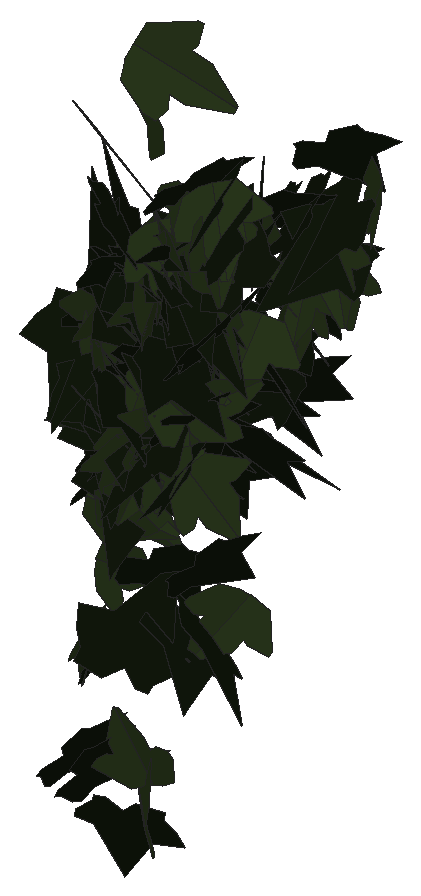
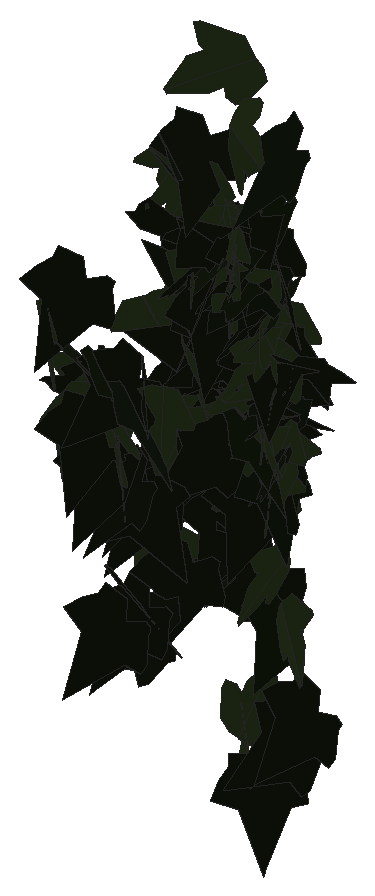
# SketchUp Ruby script. Lengths in inches.
U = 1.inch
M = Sketchup.active_model
def pt(a) = Geom::Point3d.new(a.map { |v| v * U })
def face(e, loops, mat)
  f = e.add_face(loops[0].map { |a| pt(a) })
  loops[1..].each { |l| e.add_face(l.map { |a| pt(a) }).erase! }
  f.material = f.back_material = mat if mat
  f
end
# faces: each face lists its corners as indices into pts; further lists are holes
def faces(e, pts, list, mat = nil) = list.each { |f| face(e, (f[0].is_a?(Array) ? f : [f]).map { |l| l.map { |i| pts[i] } }, mat) }
# xy, xz, yz: faces in a plane at the given z, y or x. An outline is a flat list of corners, or four numbers for a rectangle; further outlines are holes
def ring(l) = l.size == 4 ? [[l[0], l[1]], [l[2], l[1]], [l[2], l[3]], [l[0], l[3]]] : l.each_slice(2).to_a
def flat(e, list, mat, &to3) = list.each { |f| face(e, (f[0].is_a?(Array) ? f : [f]).map { |l| ring(l).map { |u, v| to3.(u, v) } }, mat) }
def xy(e, z, list, mat = nil) = flat(e, list, mat) { |x, y| [x, y, z] }
def xz(e, y, list, mat = nil) = flat(e, list, mat) { |x, z| [x, y, z] }
def yz(e, x, list, mat = nil) = flat(e, list, mat) { |y, z| [x, y, z] }
def lines(e, pts, list) = list.each { |a, b| e.add_line(pt(pts[a]), pt(pts[b])) }
# prism: a flat outline (further loops are holes) pulled along v
def prism(e, loops, v, mat = nil)
  f = face(e, loops, mat); d = Geom::Vector3d.new(v.map { |x| x * U })
  f.pushpull(f.normal.samedirection?(d) ? d.length : -d.length)
end
def box(e, o, s, mat = nil) = prism(e, [[o, [o[0] + s[0], o[1], o[2]], [o[0] + s[0], o[1] + s[1], o[2]], [o[0], o[1] + s[1], o[2]]]], [0, 0, s[2]], mat)
def at(x, y, z, deg = 0) = Geom::Transformation.translation(pt([x, y, z])) * Geom::Transformation.rotation(ORIGIN, Z_AXIS, deg.degrees)
def axes(o, x, y, z) = Geom::Transformation.new([*x, 0, *y, 0, *z, 0, *pt(o).to_a, 1])
def part(name) = M.definitions.add(name)
# library, detail: a bought-in or finely detailed component or shape, given as its bounding box
def library(name, o, s) = part(name).tap { |d| box(d.entities, o, s) }
def detail(e, o, s) = box(e.add_group.entities, o, s)
def put(e, d, t, mat = nil) = e.add_instance(d, t).tap { |i| i.material = mat if mat }
def group(e, t, mat = nil) = e.add_group.tap { |g| g.transformation = t; g.material = mat if mat }.entities
root = M.entities
M.materials.add("efeu1").color = [18, 25, 13]
M.materials.add("efeu2").color = [43, 57, 29]
c1 = part("ivyleaf_9")
p = [[1.54,2.16,1.25],[1.36,2.04,1.19],[-0.21,0.99,0.68],[-0.71,1.11,0.82],[-0.85,0.86,0.67],[-0.8,0.17,0.21],
  [-0.9,-0.01,0.1],[-0.67,-0.16,-0.02],[-0.08,-0.08,-0.05],[-0.03,-0.6,-0.4],[0.65,-0.88,-0.66],[0.83,-0.6,-0.49],
  [1.29,-0.42,-0.43],[1.8125,-0.07,-0.26],[1.21,0.44,0.15]]
faces(c1.entities,p,[[0,1,2,3,4,5,6,7,8,9,10,11,12,13,14]],"efeu1")
c2 = part("ivyleaf_10")
p = [[0,0.5,-0.03],[-0.0625,2.02,-0.43],[-0.19,2.01,-0.46],[-0.54,1.05,-0.29],[-0.52,0.625,-0.18],[-0.83,0.76,-0.28],
  [-1.16,0.64,-0.33],[-1.15,0.33,-0.24],[-0.77,-0.39,0.02],[-0.3,-0.51,0.16],[0.04,-0.48,0.23],[-0.02,2.01,-0.4375],
  [-0.06,2.01,-0.43],[0.04,-0.49,0.23],[0.67,-0.49,0.14],[1.38,0.36,-0.2],[1.375,0.51,-0.24],[0.81,0.65,-0.19],
  [0.62,0.59,-0.15],[0.6,1.09,-0.28],[0.5,1.23,-0.31]]
faces(c2.entities,p,[[0,1,2,3,4,5,6,7,8,9,10],[11,12,0,13,14,15,16,17,18,19,20]],"efeu2")
put(root,c1,axes([538.53,136.04,195.27],[-0.58778,-0.4665,-0.21206],[0.2225,0.05836,-0.74509],[0.46161,-0.62213,0.08912]))
put(root,c1,axes([538.44,141.51,191.34],[0.74287,0.20155,-0.1232],[-0.12395,-0.01349,-0.76948],[-0.20108,0.75289,0.0192]))
put(root,c1,axes([539.09,135.71,196.74],[-0.03728,0.17618,0.89989],[-0.24679,0.86548,-0.17967],[-0.88314,-0.24929,0.01222]))
put(root,c2,axes([538.71,136.07,188.61],[0.23732,-0.7524,-0.00097],[-0.00027,0.00093,-0.78894],[0.7524,0.23732,0.00002]))
put(root,c1,axes([538.61,135.22,185.86],[0.31707,0.60748,0.41139],[0.17152,0.37437,-0.68501],[-0.71334,0.36003,0.01815]))
put(root,c1,axes([538.58,142.15,191.26],[0.42447,0.59559,0.25643],[0.1387,0.216,-0.73128],[-0.63344,0.4464,0.01171]))
put(root,c2,axes([538.89,140.45,196.03],[-0.76451,-0.01451,0.16094],[-0.16108,0.00646,-0.76459],[0.01287,-0.78124,-0.00931]))
put(root,c1,axes([539.14,141.63,191.9375],[-0.73435,0.26588,-0.01109],[0.0135,0.00473,-0.78095],[-0.26577,-0.73442,-0.00904]))
put(root,c2,axes([539.02,136.29,191.62],[-0.26577,0.61137,-0.37942],[-0.14018,0.35273,0.66655],[0.70574,0.3003,-0.01048]))
put(root,c2,axes([538.94,136.37,193.18],[-0.53656,-0.52447,0.13192],[0.02393,-0.20867,-0.73229],[0.54027,-0.51162,0.16345]))
put(root,c1,axes([538.69,135.6,185.31],[0.3507,0.46919,0.5564],[0.30346,0.46711,-0.58517],[-0.66153,0.463,0.02653]))
put(root,c1,axes([538.3125,141.11,190.52],[0.67892,-0.19777,0.3143],[0.32697,0.00788,-0.70133],[0.17604,0.7481,0.09048]))
put(root,c1,axes([539.16,136,192.33],[-0.11149,0.75096,-0.08465],[0.03034,-0.08105,-0.75897],[-0.7551,-0.11413,-0.01799]))
put(root,c2,axes([538.97,136.16,189.91],[-0.06436,0.40464,0.6434],[-0.14379,0.62756,-0.40906],[-0.74634,-0.1558,0.02333]))
put(root,c2,axes([539.01,136.13,193.41],[-0.76414,0.04885,-0.02016],[0.01993,-0.00433,-0.76569],[-0.04895,-0.76439,0.00305]))
put(root,c2,axes([538.98,136.51,193.3],[0.53521,-0.53839,-0.0603],[-0.04,0.04526,-0.75914],[0.54027,0.53669,0.00353]))
put(root,c1,axes([538.66,136.36,192.97],[0.56664,-0.46286,-0.20803],[-0.16317,0.12908,-0.73165],[0.48052,0.58966,-0.00313]))
put(root,c2,axes([538.93,135.66,195.34],[-0.49499,0.55254,-0.19967],[0.0471,-0.22294,-0.73367],[-0.58562,-0.48496,0.10977]))
put(root,c1,axes([539.13,135.71,188.23],[0.06404,0.62341,0.42862],[0.0506,0.42566,-0.62667],[-0.75485,0.08142,-0.00565]))
put(root,c2,axes([539.18,136.28,193.31],[-0.29733,0.64581,-0.29043],[-0.12024,0.26438,0.71096],[0.69783,0.32072,-0.00124]))
put(root,c1,axes([539.1,136.02,195.65],[0.46406,0.52002,-0.35592],[-0.24454,-0.25876,-0.69691],[-0.58077,0.52447,0.00905]))
put(root,c1,axes([539.37,136.6875,193.67],[-0.41304,0.638,-0.06671],[0.03455,-0.0571,-0.76003],[-0.64055,-0.41448,0.00203]))
put(root,c2,axes([539.1,136.01,195.91],[0.05008,-0.78097,-0.0189],[0.00001,0.01894,-0.78257],[0.78119,0.05007,0.00122]))
put(root,c2,axes([539.01,136.07,195.71],[0.20533,0.72734,0.13381],[-0.08504,0.16117,-0.74558],[-0.73464,0.18463,0.1237]))
put(root,c2,axes([539.28,135.55,195.97],[-0.77005,-0.09821,0.12045],[-0.11673,-0.03643,-0.776],[0.1026,-0.77856,0.02112]))
put(root,c1,axes([539.16,136.36,191.87],[0.43792,0.62601,-0.00664],[-0.04534,0.02363,-0.76229],[-0.6244,0.43733,0.05069]))
put(root,c1,axes([539.5,140.52,193.58],[0.18787,0.37763,-0.67113],[-0.36275,-0.56598,-0.42001],[-0.67929,0.40668,0.03867]))
put(root,c1,axes([539.57,140.54,195.95],[-0.40924,0.64709,0.05819],[-0.05149,0.03625,-0.76527],[-0.64766,-0.41177,0.02407]))
put(root,c1,axes([539.34,136.1,184.42],[0.4741,0.4396,-0.42175],[-0.32938,-0.2646,-0.64606],[-0.51247,0.57675,0.02506]))
put(root,c2,axes([538.93,136.23,195.36],[-0.51058,-0.24186,-0.52391],[0.48664,0.19546,-0.56449],[0.3101,-0.70496,0.02323]))
put(root,c2,axes([539.46,135.99,196.65],[0.65655,0.0303,0.42722],[-0.42516,0.14055,0.64341],[-0.05173,-0.7706,0.13415]))
put(root,c1,axes([539.1875,138.96,191.11],[0.58178,0.45882,-0.17486],[-0.14194,-0.10238,-0.7409],[-0.47005,0.5988,0.0073]))
put(root,c2,axes([539.375,136.34,192.25],[-0.59922,-0.4744,0.03321],[-0.01406,-0.03573,-0.76404],[0.47535,-0.59908,0.01927]))
put(root,c1,axes([539.57,140,195.3],[0.03019,-0.03122,0.78694],[-0.059,0.78521,0.03341],[-0.78534,-0.06019,0.02774]))
put(root,c1,axes([538.76,136,193.32],[0.49045,-0.46614,0.3861],[0.32311,-0.21857,-0.67433],[0.51181,0.58467,0.05573]))
put(root,c1,axes([539.08,140.93,194.15],[0.73449,-0.11145,-0.17675],[-0.1718,0.04555,-0.74266],[0.11893,0.75409,0.01873]))
put(root,c1,axes([539.24,136.27,193.3125],[-0.31359,-0.68107,-0.16899],[0.06083,0.15802,-0.74972],[0.69908,-0.31926,-0.01057]))
put(root,c1,axes([539.1,135.79,194.33],[-0.2288,-0.619,-0.39012],[0.23384,0.32545,-0.65353],[0.6933,-0.31405,0.09168]))
put(root,c1,axes([539.07,135.43,200.25],[0.77153,-0.18345,-0.19129],[-0.179,0.07354,-0.7925],[0.19546,0.79148,0.0293]))
put(root,c1,axes([539.16,136.35,193.6],[0.15372,-0.74823,0.02172],[0.01041,-0.02003,-0.76384],[0.74848,0.15395,0.00616]))
put(root,c1,axes([539.8,135.85,197.48],[0.14738,-0.27916,0.7209],[-0.28426,0.6629,0.31481],[-0.71891,-0.31935,0.02331]))
put(root,c1,axes([540.0625,136.15,193.84],[-0.62363,0.07895,0.4451],[-0.45146,-0.07016,-0.62009],[-0.02302,-0.76296,0.10308]))
put(root,c1,axes([539.5,135.76,192.64],[0.54446,0.52606,-0.19868],[-0.14023,-0.14079,-0.75708],[-0.54456,0.56222,-0.00368]))
put(root,c1,axes([539.1,136,194.69],[0.67186,-0.36722,0.05072],[0.04461,-0.02414,-0.76566],[0.36801,0.67334,0.00021]))
put(root,c2,axes([539.55,136.29,194.39],[0.3664,0.66496,-0.11623],[-0.06535,-0.09668,-0.75915],[-0.67187,0.37203,0.01046]))
put(root,c2,axes([540.16,135.96,200.58],[0.0647,0.16542,-0.9116],[-0.60391,0.70055,0.08426],[0.70262,0.58689,0.15636]))
put(root,c2,axes([539.9,136.06,185.58],[-0.71595,-0.1147,-0.27326],[-0.27033,-0.04006,0.72507],[-0.12145,0.76528,-0.00301]))
put(root,c2,axes([539.77,135.75,193.06],[-0.11188,-0.77393,0.12518],[-0.03611,-0.12123,-0.78176],[0.78316,-0.11615,-0.01817]))
put(root,c1,axes([539.53,135.26,198.58],[0.66555,-0.11445,-0.45218],[-0.39862,0.26955,-0.65496],[0.2422,0.75814,0.1646]))
put(root,c1,axes([539.18,135.93,196.33],[0.5444,-0.56867,-0.01587],[0.08546,0.10348,-0.77588],[0.56243,0.53471,0.13327]))
put(root,c1,axes([539.57,136.26,192.18],[-0.27136,-0.71818,0.01274],[-0.00829,-0.01048,-0.76772],[0.71824,-0.27145,-0.00404]))
put(root,c1,axes([539.43,135.86,194.3],[0.41124,-0.62924,-0.14894],[-0.09481,0.11593,-0.75154],[0.63964,0.42174,-0.01563]))
put(root,c2,axes([539.24,135.71,191.61],[-0.21709,-0.05124,-0.74696],[0.74868,-0.00786,-0.21705],[0.00673,-0.77782,0.0514]))
put(root,c2,axes([539.94,140.44,194.36],[0.27835,-0.63522,-0.39024],[-0.12857,0.36941,-0.69302],[0.73435,0.30545,0.02658]))
put(root,c1,axes([539.53,136.18,195.97],[0.14442,-0.7539,-0.09451],[-0.00127,0.09596,-0.76743],[0.7598,0.14346,0.01668]))
put(root,c2,axes([540.32,135.65,184.79],[-0.04086,0.03215,0.85887],[-0.72205,0.46511,-0.05176],[-0.46619,-0.72319,0.00489]))
put(root,c1,axes([539.64,140.38,196.36],[0.60017,0.42917,0.21801],[0.14139,0.1759,-0.73551],[-0.46013,0.61383,0.05835]))
put(root,c1,axes([540,135.28,197.6],[0.26048,0.73966,-0.10409],[-0.02755,-0.10064,-0.78415],[-0.74644,0.26183,-0.00738]))
put(root,c1,axes([539.83,140.85,194.46],[0.57492,0.49964,-0.08552],[-0.06595,-0.05449,-0.76169],[-0.50259,0.57869,0.00212]))
put(root,c1,axes([539.57,135.66,197.24],[0.7954,0.06777,-0.01492],[-0.01803,0.03606,-0.7974],[-0.06701,0.79472,0.03745]))
put(root,c1,axes([539.76,139.7,193.59],[0.70856,-0.13217,-0.26729],[-0.2648,0.03793,-0.72071],[0.1371,0.75635,-0.01057]))
put(root,c2,axes([540.15,140.76,194.43],[-0.69774,0.29461,0.11061],[-0.16794,-0.12109,-0.73689],[-0.26613,-0.696,0.17502]))
put(root,c2,axes([540.08,135.84,193.73],[-0.37993,-0.67566,-0.15848],[0.08193,0.13574,-0.77514],[0.68915,-0.38863,0.00479]))
put(root,c2,axes([540.0625,136.17,192.79],[0.10105,0.5459,-0.5384],[-0.15888,-0.51636,-0.55337],[-0.75009,0.18292,0.04468]))
put(root,c2,axes([540.17,136.16,192.92],[-0.0825,-0.7681,-0.05601],[0.00594,0.05569,-0.77252],[0.77012,-0.08271,-0.00004]))
put(root,c2,axes([539.86,135.58,192.05],[-0.60774,-0.1913,-0.45576],[0.43367,0.14021,-0.63713],[0.23717,-0.7466,-0.00287]))
put(root,c1,axes([540.51,140.49,196.55],[-0.53165,0.55634,-0.04476],[0.02945,-0.03377,-0.76952],[-0.55736,-0.53247,0.00204]))
put(root,c1,axes([539.77,137.02,193.14],[0.73656,0.16562,0.11181],[0.10375,0.048,-0.75458],[-0.17078,0.74345,0.02381]))
put(root,c1,axes([539.95,135.43,188.34],[-0.52,-0.0198,0.64991],[0.64749,-0.09172,0.51527],[0.05934,0.82726,0.07268]))
put(root,c2,axes([540.2,135.89,195.25],[0.73426,-0.18056,-0.13904],[-0.12838,0.05984,-0.75565],[0.18829,0.74491,0.027]))
put(root,c1,axes([539.71,136.0625,192.59],[0.641,0.10651,0.41568],[0.41518,0.03491,-0.64918],[-0.10845,0.76319,-0.02832]))
put(root,c2,axes([540.35,135.8,196.75],[-0.14563,-0.7749,-0.08204],[0.00751,0.08206,-0.78843],[0.7792,-0.14562,-0.00773]))
put(root,c1,axes([539.82,135.71,194.96],[0.65321,0.16006,0.40835],[0.36604,0.20462,-0.66573],[-0.24163,0.74267,0.09542]))
put(root,c2,axes([540.56,135.81,197.4375],[-0.52433,0.42473,0.41549],[-0.34106,0.23859,-0.67431],[-0.48651,-0.625,0.02494]))
put(root,c2,axes([540.48,136.11,193.27],[-0.72373,0.27178,0.07148],[-0.16863,-0.26201,-0.71111],[-0.22481,-0.67841,0.30328]))
put(root,c2,axes([540.3,136.01,197.1],[0.48381,-0.55944,-0.23219],[0.02325,0.3141,-0.70835],[0.60526,0.43511,0.21281]))
put(root,c1,axes([540.52,135.98,193.61],[-0.73143,0.00939,-0.24476],[0.23938,-0.1359,-0.72056],[-0.05189,-0.75923,0.12595]))
put(root,c1,axes([540.39,140.87,195.26],[0.34958,0.6864,-0.0181],[-0.01771,-0.01129,-0.77022],[-0.68641,0.34987,0.01066]))
put(root,c1,axes([540.13,136.08,196.84],[-0.02439,-0.76512,-0.14188],[-0.00251,0.14203,-0.76548],[0.77816,-0.02353,-0.00692]))
put(root,c2,axes([540.3,140.61,194.98],[0.75681,-0.14576,-0.01688],[-0.00701,0.05269,-0.76907],[0.14657,0.75516,0.0504]))
put(root,c1,axes([539.86,135.89,196.98],[0.70136,-0.35616,0.06992],[0.15876,0.16424,-0.75595],[0.32639,0.68543,0.21747]))
put(root,c1,axes([540.37,135.73,190.65],[0.53379,0.55048,-0.02803],[-0.01899,-0.02063,-0.76678],[-0.55087,0.53412,-0.00073]))
put(root,c2,axes([540.42,136.8,193.61],[0.55388,0.50607,-0.15458],[-0.10823,-0.1107,-0.75021],[-0.51796,0.56429,-0.00854]))
put(root,c1,axes([540.62,136.14,196.125],[0.16222,0.75869,0.02151],[0.00731,0.02043,-0.77583],[-0.75896,0.16236,-0.00288]))
put(root,c2,axes([540.72,135,196.52],[-0.01675,0.15895,-0.81027],[-0.14412,0.79743,0.15942],[0.81304,0.14462,0.01156]))
put(root,c2,axes([540.7,135.95,197.89],[-0.769,0.14951,0.08378],[-0.10546,-0.1092,-0.7731],[-0.13509,-0.76581,0.1266]))
put(root,c1,axes([540.26,136.17,195.48],[0.84849,0.08014,0.01658],[0.01652,0.00137,-0.85226],[-0.08015,0.84865,-0.00019]))
put(root,c2,axes([540.68,140.57,195.51],[-0.74273,-0.18107,-0.11001],[0.10641,0.02801,-0.76448],[0.18321,-0.75031,-0.00199]))
put(root,c1,axes([540.48,138.47,192.33],[0.72105,0.23572,-0.12573],[-0.13083,-0.00395,-0.75773],[-0.23293,0.73192,0.0364]))
put(root,c1,axes([540.96,135.76,197.87],[-0.00501,0.6946,-0.36013],[-0.10903,-0.35724,-0.68752],[-0.77478,0.04578,0.09908]))
put(root,c2,axes([540.61,135.8,198.06],[-0.57939,0.52515,-0.13268],[0.08864,-0.09973,-0.78184],[-0.53435,-0.58597,0.01416]))
put(root,c2,axes([540.86,140.86,195.22],[-0.75873,-0.1281,-0.03694],[0.03399,0.02052,-0.76933],[0.12891,-0.75935,-0.01456]))
put(root,c1,axes([541.21,135.81,193.08],[-0.52854,0.55938,-0.10568],[0.05434,-0.09397,-0.76918],[-0.56668,-0.53074,0.02481]))
put(root,c2,axes([540.7,135.59,198.08],[0.39838,0.67987,0.10779],[0.05605,0.09209,-0.78799],[-0.68608,0.4023,-0.00178]))
put(root,c2,axes([540.94,136.07,193.79],[0.10231,0.76287,-0.12227],[0.02302,0.12027,0.76967],[0.77226,-0.10465,-0.00674]))
put(root,c1,axes([540.85,135.875,196.76],[0.4965,-0.37139,-0.5915],[-0.48138,0.34385,-0.61996],[0.50604,0.69149,-0.0094]))
put(root,c1,axes([540.6,136.61,188.73],[-0.0334,-0.68806,0.37792],[0.1855,-0.37447,-0.66538],[0.76279,0.06094,0.17836]))
put(root,c2,axes([541,136.71,194.88],[0.55212,-0.53266,-0.05984],[-0.0449,0.03965,-0.76717],[0.53413,0.55393,-0.00263]))
put(root,c1,axes([540.54,136.06,197.35],[0.57869,-0.50888,-0.1274],[0.0377,0.22954,-0.74563],[0.52323,0.54628,0.19463]))
put(root,c1,axes([541.3,140.6875,196.03],[-0.63364,-0.37236,0.2477],[-0.15688,-0.21719,-0.72782],[0.4188,-0.64473,0.10213]))
put(root,c1,axes([540.52,136.21,194.82],[0.30174,-0.02511,0.70963],[0.70009,0.13936,-0.29275],[-0.11866,0.75842,0.07728]))
put(root,c2,axes([540.49,135.61,202.13],[0.33124,0.25516,0.83214],[0.64185,0.52977,-0.41793],[-0.58788,0.72217,0.01257]))
put(root,c2,axes([541.29,135.61,198.89],[0.57767,-0.36469,-0.40185],[-0.29485,0.2818,-0.67959],[0.45558,0.64481,0.06972]))
put(root,c1,axes([541.16,136.04,194.08],[0.30095,0.71932,-0.04549],[-0.01052,-0.04491,-0.7797],[-0.72068,0.30104,-0.00761]))
put(root,c1,axes([540.91,135.91,197.73],[-0.2262,-0.56696,-0.49776],[0.28679,0.41603,-0.6042],[0.69783,-0.35476,0.08696]))
put(root,c2,axes([541.34,135.67,198.02],[-0.77811,-0.06881,0.01909],[-0.01939,0.00248,-0.78114],[0.06873,-0.77834,-0.00418]))
put(root,c1,axes([541.41,140.78,196.85],[-0.72209,-0.00151,-0.28626],[0.27474,-0.22191,-0.69184],[-0.08044,-0.74439,0.20683]))
put(root,c1,axes([541.14,140.36,198.35],[0.54956,0.5533,0.00685],[0.01137,-0.00163,-0.77979],[-0.55323,0.5496,-0.00921]))
put(root,c1,axes([541.05,135.42,195.92],[0.28418,-0.53431,-0.57149],[-0.24901,0.51463,-0.60498],[0.74168,0.37751,0.01586]))
put(root,c1,axes([541.48,135.4375,199.74],[0.22993,0.77216,0.09879],[-0.04886,0.11712,-0.80172],[-0.77692,0.22116,0.07965]))
put(root,c2,axes([541.03,140.45,195.96],[0.72751,0.02287,0.33345],[0.33215,0.03971,-0.72739],[-0.03732,0.7993,0.0266]))
put(root,c2,axes([541.76,136.66,189.64],[0.56743,0.32209,-0.44924],[-0.48732,-0.01239,-0.62442],[-0.26091,0.72363,0.18927]))
put(root,c1,axes([541.1875,136.08,196.83],[0.27243,-0.66723,-0.29761],[-0.00805,0.31487,-0.71329],[0.73055,0.25229,0.10313]))
put(root,c1,axes([542.16,136.21,197.39],[-0.13371,0.26172,0.72516],[-0.71704,0.22815,-0.21455],[-0.28321,-0.7012,0.20086]))
put(root,c2,axes([541.1875,136.05,194.17],[-0.3558,-0.29774,0.62876],[0.48199,0.40376,0.46395],[-0.50167,0.59909,-0.00019]))
put(root,c2,axes([541.44,135.84,192.72],[0.21816,0.6149,0.42528],[0.07482,0.42283,-0.64975],[-0.74389,0.22287,0.05937]))
put(root,c2,axes([541.45,136.42,196.63],[-0.56721,0.38595,-0.36474],[0.26645,-0.25479,-0.68396],[-0.45934,-0.62438,0.05364]))
put(root,c1,axes([541.4,135.52,195.5625],[0.08294,0.78143,0.02976],[-0.00303,-0.0296,0.78582],[0.782,-0.083,-0.00011]))
put(root,c2,axes([541.91,140.83,197.35],[0.46024,-0.48565,-0.40345],[-0.20851,0.35434,-0.6644],[0.59595,0.49904,0.07912]))
put(root,c1,axes([541.22,136.3125,189.15],[0.35478,-0.65507,0.41288],[0.21998,-0.35018,-0.74461],[0.74243,0.41679,0.02332]))
put(root,c1,axes([542.14,135.65,199.5],[-0.55109,0.57058,-0.09539],[0.0563,-0.07822,-0.79314],[-0.57575,-0.55379,0.01374]))
put(root,c1,axes([541.79,135.375,191.21],[0.32125,0.65505,0.26755],[0.1203,0.23899,-0.72958],[-0.69729,0.34303,-0.00261]))
put(root,c1,axes([542.43,135.72,198.89],[-0.67213,0.3991,0.09668],[-0.11239,-0.00043,-0.77958],[-0.39496,-0.67905,0.05732]))
put(root,c2,axes([542.01,136.88,195.9],[0.56554,0.46383,-0.26625],[-0.22457,-0.14573,-0.73088],[-0.48538,0.60785,0.02794]))
put(root,c2,axes([541.96,135.72,198.72],[0.07813,0.78127,-0.03035],[-0.03822,-0.02665,-0.78437],[-0.78092,0.07947,0.03535]))
put(root,c2,axes([541.99,135.67,199.35],[0.50138,0.59568,0.11552],[0.06881,0.09307,-0.77857],[-0.60287,0.50602,0.00721]))
